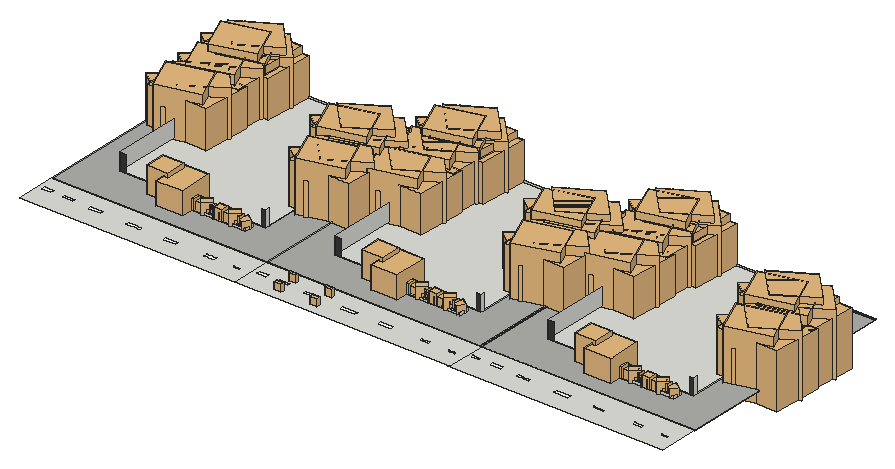
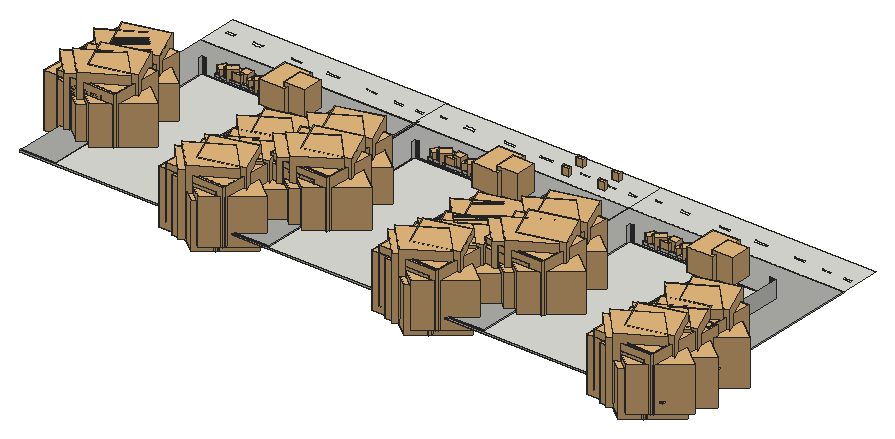
# SketchUp Ruby script. Lengths in inches.
U = 1.inch
M = Sketchup.active_model
def pt(a) = Geom::Point3d.new(a.map { |v| v * U })
def face(e, loops, mat)
  f = e.add_face(loops[0].map { |a| pt(a) })
  loops[1..].each { |l| e.add_face(l.map { |a| pt(a) }).erase! }
  f.material = f.back_material = mat if mat
  f
end
# faces: each face lists its corners as indices into pts; further lists are holes
def faces(e, pts, list, mat = nil) = list.each { |f| face(e, (f[0].is_a?(Array) ? f : [f]).map { |l| l.map { |i| pts[i] } }, mat) }
# xy, xz, yz: faces in a plane at the given z, y or x. An outline is a flat list of corners, or four numbers for a rectangle; further outlines are holes
def ring(l) = l.size == 4 ? [[l[0], l[1]], [l[2], l[1]], [l[2], l[3]], [l[0], l[3]]] : l.each_slice(2).to_a
def flat(e, list, mat, &to3) = list.each { |f| face(e, (f[0].is_a?(Array) ? f : [f]).map { |l| ring(l).map { |u, v| to3.(u, v) } }, mat) }
def xy(e, z, list, mat = nil) = flat(e, list, mat) { |x, y| [x, y, z] }
def xz(e, y, list, mat = nil) = flat(e, list, mat) { |x, z| [x, y, z] }
def yz(e, x, list, mat = nil) = flat(e, list, mat) { |y, z| [x, y, z] }
def lines(e, pts, list) = list.each { |a, b| e.add_line(pt(pts[a]), pt(pts[b])) }
# prism: a flat outline (further loops are holes) pulled along v
def prism(e, loops, v, mat = nil)
  f = face(e, loops, mat); d = Geom::Vector3d.new(v.map { |x| x * U })
  f.pushpull(f.normal.samedirection?(d) ? d.length : -d.length)
end
def box(e, o, s, mat = nil) = prism(e, [[o, [o[0] + s[0], o[1], o[2]], [o[0] + s[0], o[1] + s[1], o[2]], [o[0], o[1] + s[1], o[2]]]], [0, 0, s[2]], mat)
def at(x, y, z, deg = 0) = Geom::Transformation.translation(pt([x, y, z])) * Geom::Transformation.rotation(ORIGIN, Z_AXIS, deg.degrees)
def axes(o, x, y, z) = Geom::Transformation.new([*x, 0, *y, 0, *z, 0, *pt(o).to_a, 1])
def part(name) = M.definitions.add(name)
# library, detail: a bought-in or finely detailed component or shape, given as its bounding box
def library(name, o, s) = part(name).tap { |d| box(d.entities, o, s) }
def detail(e, o, s) = box(e.add_group.entities, o, s)
def put(e, d, t, mat = nil) = e.add_instance(d, t).tap { |i| i.material = mat if mat }
def group(e, t, mat = nil) = e.add_group.tap { |g| g.transformation = t; g.material = mat if mat }.entities
root = M.entities
M.materials.add("Color_000").color = [255, 255, 255]
M.materials.add("Material__1").color = [95, 70, 46]
M.materials.add("[Color M07]").color = [58, 58, 58]
M.materials.add("[Concrete Block 8x8 Gray]").color = [177, 178, 173]
M.materials.add("[Wood Veneer 01]").color = [120, 70, 37]
c1 = library("Group\#46",[-33.32,-34.9375,32.67],[162.87,159.66,128.34])
c2 = library("Group\#62",[-10.45,-6.67,0],[121.7,116.61,164.95])
c3 = library("Group\#64",[-10.45,-6.67,0],[121.7,116.61,164.95])
c4 = library("Group\#47",[-10.45,-6.67,0],[121.7,116.61,164.95])
c5 = library("Group\#65",[-33.32,-34.9375,32.67],[162.87,159.66,128.34])
c6 = library("Group\#45",[-33.32,-34.9375,81.35],[162.87,159.66,79.66])
c7 = library("Group\#57",[-33.32,-34.9375,77.91],[162.87,159.66,83.1])
c8 = part("Palem Elek")
put(c8.entities,c1,axes([92.2,20.3,-29.73],[0.70711,0.70711,0],[-0.70711,0.70711,0],[0,0,0.91208]))
put(c8.entities,c2,axes([60.27,20.78,0],[1,0,0],[0,1,0],[0,0,0.85762]))
put(c8.entities,c3,at(25.45,60.83,0,-53.5))
put(c8.entities,c4,at(84.4375,135.48,0,-161.4))
put(c8.entities,c5,axes([38.54,105.7,-36.19],[-0.04013,-0.99919,0],[0.99919,-0.04013,0],[0,0,1.11001]))
put(c8.entities,c6,axes([57.15,96.51,-54.45],[-0.02003,-0.49872,0.02965],[0.4996,-0.02007,0],[0.00123,0.03065,0.51628]))
put(c8.entities,c7,axes([74.94,50.39,-54.06],[0.40095,0.29715,0.03075],[-0.29654,0.38966,0.10114],[0.04012,-0.11026,0.54246]))
c9 = part("palem elek\#1")
put(c9.entities,c8,at(-81.14,-74.56,-0.83))
c10 = part("Coqueiro")
put(c10.entities,c9,axes([83.17,89.39,9.5625],[0,1.1016,0],[-1.377,0,0],[0,0,1.39284]))
c11 = library("Areca palm plant",[0,0,0],[49.1,36.6,54.46])
c12 = library("Group\#130",[-7.34,-1.2,0],[38.67,35.81,49.04])
c13 = library("Group\#74",[-84.69,-90.07,-0.36],[176.51,175.13,171.4])
c14 = library("Group38\#2",[14.01,28.44,-23.43],[18.58,18.32,38.89])
c15 = library("Group20\#1",[-20.81,-17.08,3.79],[39.86,39.43,37.51])
c16 = part("Group\#6")
put(c16.entities,c11,axes([-6.2,158.41,6.08],[0.45017,-0.56191,0],[0.66137,0.52986,0],[0,0,0.72]))
put(c16.entities,c11,axes([-6.2,56.6,6.08],[0.45017,-0.56191,0],[0.66137,0.52986,0],[0,0,0.72]))
put(c16.entities,c12,axes([24.9375,191.72,8],[0,0.79,0],[-0.79,0,0],[0,0,0.79]))
put(c16.entities,c13,axes([14.93,91.37,6.05],[-0.04961,-0.08593,0],[0.08593,-0.04961,0],[0,0,0.10522]))
put(c16.entities,c13,axes([17.19,15.79,6.07],[-0.08133,-0.14087,0],[0.14087,-0.08133,0],[0,0,0.1725]))
put(c16.entities,c13,axes([17.19,223.04,6.07],[-0.08133,-0.14087,0],[0.14087,-0.08133,0],[0,0,0.1725]))
put(c16.entities,c13,axes([17.19,121.23,6.07],[-0.08133,-0.14087,0],[0.14087,-0.08133,0],[0,0,0.1725]))
put(c16.entities,c13,axes([14.93,145.87,6.05],[-0.04961,-0.08593,0],[0.08593,-0.04961,0],[0,0,0.10522]))
put(c16.entities,c12,axes([24.9375,89.91,8],[0,0.79,0],[-0.79,0,0],[0,0,0.79]))
put(c16.entities,c14,axes([-4.1,-1.15,28.17],[0.8848,0,0],[0,0.94674,0],[0,0,0.85826]))
put(c16.entities,c13,axes([14.93,44.05,6.05],[-0.04961,-0.08593,0],[0.08593,-0.04961,0],[0,0,0.10522]))
put(c16.entities,c13,axes([14.93,193.18,6.05],[-0.04961,-0.08593,0],[0.08593,-0.04961,0],[0,0,0.10522]))
put(c16.entities,c13,axes([14.93,71.3,6.05],[-0.04961,-0.08593,0],[0.08593,-0.04961,0],[0,0,0.10522]))
put(c16.entities,c13,axes([14.93,173.12,6.05],[-0.04961,-0.08593,0],[0.08593,-0.04961,0],[0,0,0.10522]))
put(c16.entities,c15,axes([18.97,79.98,4.77],[0,0.85,0],[-0.85,0,0],[0,0,0.85]))
g1 = group(c16.entities,at(0,0,0))
xy(g1,0,[[0,0,6,234.8],[30,0,36,234.8]])
xy(g1,3,[[6,0,30,234.8]])
xy(g1,7,[[6,5,30,229.8]],"Material__1")
xy(g1,15,[[[0,0,36,234.8],[6,5,30,229.8]]])
xz(g1,0,[[0,0,6,0,6,3,30,3,30,0,36,0,36,15,0,15]])
xz(g1,5,[[6,7,30,15]])
xz(g1,229.8,[[6,7,30,15]])
xz(g1,234.8,[[0,0,0,15,36,15,36,0,30,0,30,3,6,3,6,0]])
yz(g1,0,[[0,0,234.8,15]])
yz(g1,6,[[0,0,234.8,3],[5,7,229.8,15]])
yz(g1,30,[[0,0,234.8,3],[5,7,229.8,15]])
yz(g1,36,[[0,0,234.8,15]])
put(c16.entities,c14,axes([-4.1,100.66,28.17],[0.8848,0,0],[0,0.94674,0],[0,0,0.85826]))
put(c16.entities,c15,axes([18.97,181.79,4.77],[0,0.85,0],[-0.85,0,0],[0,0,0.85]))
c17 = library("Sem+nome (1)",[20.77,3.52,-2.22],[96.42,122.82,82.56])
c18 = library("Pot+Plant",[-20.81,-17.08,-0.03],[39.86,39.43,41.33])
c19 = part("Untitled (5)")
xy(c19.entities,0,[[[158.81,26.5625,306.06,993.3125],[226.57,518.17,239.57,583.92],[225.28,357.51,237.28,411.51],[222.61,182.28,236.36,226.53],[239.71,931.55,251.46,972.3],[233.64,703.93,242.14,755.18],[240.05,835.03,248.8,880.53],[222.04,66.5,231.29,100.5]]])
xy(c19.entities,0,[[222.04,66.5,231.29,100.5],[222.61,182.28,236.36,226.53],[225.28,357.51,237.28,411.51],[226.57,518.17,239.57,583.92],[233.64,703.93,242.14,755.18],
  [240.05,835.03,248.8,880.53],[239.71,931.55,251.46,972.3]],"Color_000")
c20 = library("Car wheel",[-30.53,-13.73,-29.67],[182.47,72.82,182.83])
c21 = library("Floor plant",[-5.56,-16.3125,0.81],[76.88,76.71,92.33])
xy(root,0,[[674.46,147.25,1460.84,975.9375],[1460.84,147.25,2241.21,975.9375],[2241.21,147.25,2247.21,975.9375],[2247.21,147.25,3027.59,975.9375]])
xy(root,3.54,[[674.46,147.25,1460.84,147.25,1460.84,969.375,1334.59,969.375,1334.59,301,800.71,301,800.71,975.9375,674.46,975.9375],[1460.84,147.25,2241.21,147.25,2241.21,969.375,2120.96,969.375,2120.96,301,1587.09,301,1587.09,975.9375,1460.84,975.9375],[2241.21,147.25,2247.21,969.375],[2247.21,147.25,3027.59,147.25,3027.59,969.375,2901.34,969.375,2901.34,301,2367.46,301,2367.46,975.9375,2241.21,975.9375,2241.21,969.375,2247.21,969.375]],"[Concrete Block 8x8 Gray]")
xz(root,147.25,[[674.46,0,1460.84,3.54],[1460.84,0,2241.21,3.54],[2241.21,0,2247.21,3.54],[2247.21,0,3027.59,3.54]])
xz(root,301,[[800.71,3.54,1334.59,3.54,1334.59,62.25,1320.28,62.25,1320.28,54.66,1320.57,54.66,1320.57,5.875,998.26,5.875,998.26,65.875,982.13,65.875,982.13,5.875,823.45,5.875,823.45,65.875,800.71,65.875],[1587.09,3.54,2120.96,3.54,2120.96,62.25,2106.65,62.25,2106.65,54.66,2106.94,54.66,2106.94,5.875,1784.63,5.875,1784.63,65.875,1768.51,65.875,1768.51,5.875,1609.83,5.875,1609.83,65.875,1587.09,65.875],[2367.46,3.54,2901.34,3.54,2901.34,62.25,2887.03,62.25,2887.03,54.66,2887.32,54.66,2887.32,5.875,2565.01,5.875,2565.01,65.875,2548.88,65.875,2548.88,5.875,2390.2,5.875,2390.2,65.875,2367.46,65.875]],"[Color M07]")
xz(root,969.375,[[1334.59,3.54,1460.84,5.875],[2120.96,3.54,2247.21,5.875],[2901.34,3.54,3027.59,5.875]])
xz(root,975.9375,[[674.46,0,674.46,3.54,800.71,3.54,800.71,65.875,874.71,65.875,874.71,5.875,1460.84,5.875,1460.84,0],[1460.84,0,1460.84,3.54,1587.09,3.54,1587.09,65.875,1661.09,65.875,1661.09,5.875,2247.21,5.875,2247.21,3.54,2241.21,3.54,2241.21,0],[2241.21,0,2247.21,3.54],[2247.21,0,2247.21,3.54,2367.46,3.54,2367.46,65.875,2441.46,65.875,2441.46,5.875,3027.59,5.875,3027.59,0]])
yz(root,674.46,[[147.25,0,975.9375,3.54]])
yz(root,800.71,[[301,3.54,975.9375,65.875]])
yz(root,1334.59,[[301,3.54,315.3125,62.25],[315.3125,3.54,969.375,5.875]])
yz(root,1460.84,[[147.25,0,975.9375,3.54],[969.375,3.54,975.9375,5.875]])
yz(root,1587.09,[[301,3.54,975.9375,65.875]])
yz(root,2120.96,[[301,3.54,315.3125,62.25],[315.3125,3.54,969.375,5.875]])
yz(root,2241.21,[[147.25,0,975.9375,3.54]])
yz(root,2247.21,[[147.25,0,975.9375,0,975.9375,5.875,969.375,5.875,969.375,3.54,147.25,3.54]])
yz(root,2367.46,[[301,3.54,975.9375,65.875]])
yz(root,2901.34,[[301,3.54,315.3125,62.25],[315.3125,3.54,969.375,5.875]])
yz(root,3027.59,[[969.375,3.54,975.9375,5.875]])
put(root,c10,at(1509.73,805.4,-72.06))
put(root,c10,at(1483.35,700.96,-72.06))
put(root,c10,at(1483.35,554.77,-72.06))
put(root,c10,at(696.98,554.77,-72.06))
put(root,c10,at(723.35,805.4,-72.06))
put(root,c10,at(696.98,700.96,-72.06))
put(root,c10,at(2263.73,554.77,-72.06))
put(root,c10,at(2290.1,805.4,-72.06))
put(root,c10,at(2263.73,700.96,-72.06))
put(root,c10,at(2094.23,599.81,-52.61))
put(root,c10,at(2094.23,444.18,-52.61))
put(root,c10,at(1307.86,599.81,-52.61))
put(root,c10,at(1307.86,444.18,-52.61))
put(root,c10,at(2874.61,444.18,-52.61))
put(root,c10,at(2874.61,599.81,-52.61))
put(root,c10,at(1484.12,805.15,-48.82))
put(root,c10,at(697.74,805.15,-48.82))
put(root,c10,at(2264.49,805.15,-48.82))
put(root,c10,at(2046.73,599.81,-31.76))
put(root,c10,at(1260.36,599.81,-31.76))
put(root,c10,at(2827.11,599.81,-31.76))
put(root,c16,at(2085.11,251.93,-3.46,90))
put(root,c16,at(1298.73,251.93,-3.46,90))
put(root,c16,at(2865.48,251.93,-3.46,90))
put(root,c17,at(1770.51,206.86,3.54),"[Wood Veneer 01]")
put(root,c17,at(984.13,206.86,3.54),"[Wood Veneer 01]")
put(root,c17,at(2550.88,206.86,3.54),"[Wood Veneer 01]")
put(root,c18,at(1793.03,287.15,3.54))
put(root,c18,at(1006.66,287.15,3.54))
put(root,c18,at(2573.41,287.15,3.54))
put(root,c19,axes([2268.82,-158.81,3.54],[0,1,0],[-0.81342,0,0],[0,0,1]))
put(root,c20,axes([1712.58,112.21,7.77],[0.14273,0,0],[0,-0.16112,0],[0,0,0.14273]))
put(root,c20,axes([1712.58,38.19,7.77],[0.14273,0,0],[0,0.16112,0],[0,0,0.14273]))
put(root,c19,axes([1482.45,-158.81,3.54],[0,1,0],[-0.81342,0,0],[0,0,1]))
put(root,c19,axes([3049.2,-158.81,3.54],[0,1,0],[-0.81342,0,0],[0,0,1]))
put(root,c20,axes([1580.34,38.39,8.09],[0.14273,0,0],[0,0.16112,0],[0,0,0.14273]))
put(root,c20,axes([1580.34,112.01,8.09],[0.14273,0,0],[0,-0.16112,0],[0,0,0.14273]))
put(root,c21,at(1734.67,260.95,3.54))
put(root,c21,at(948.3,260.95,3.54))
put(root,c21,at(2515.05,260.95,3.54))
